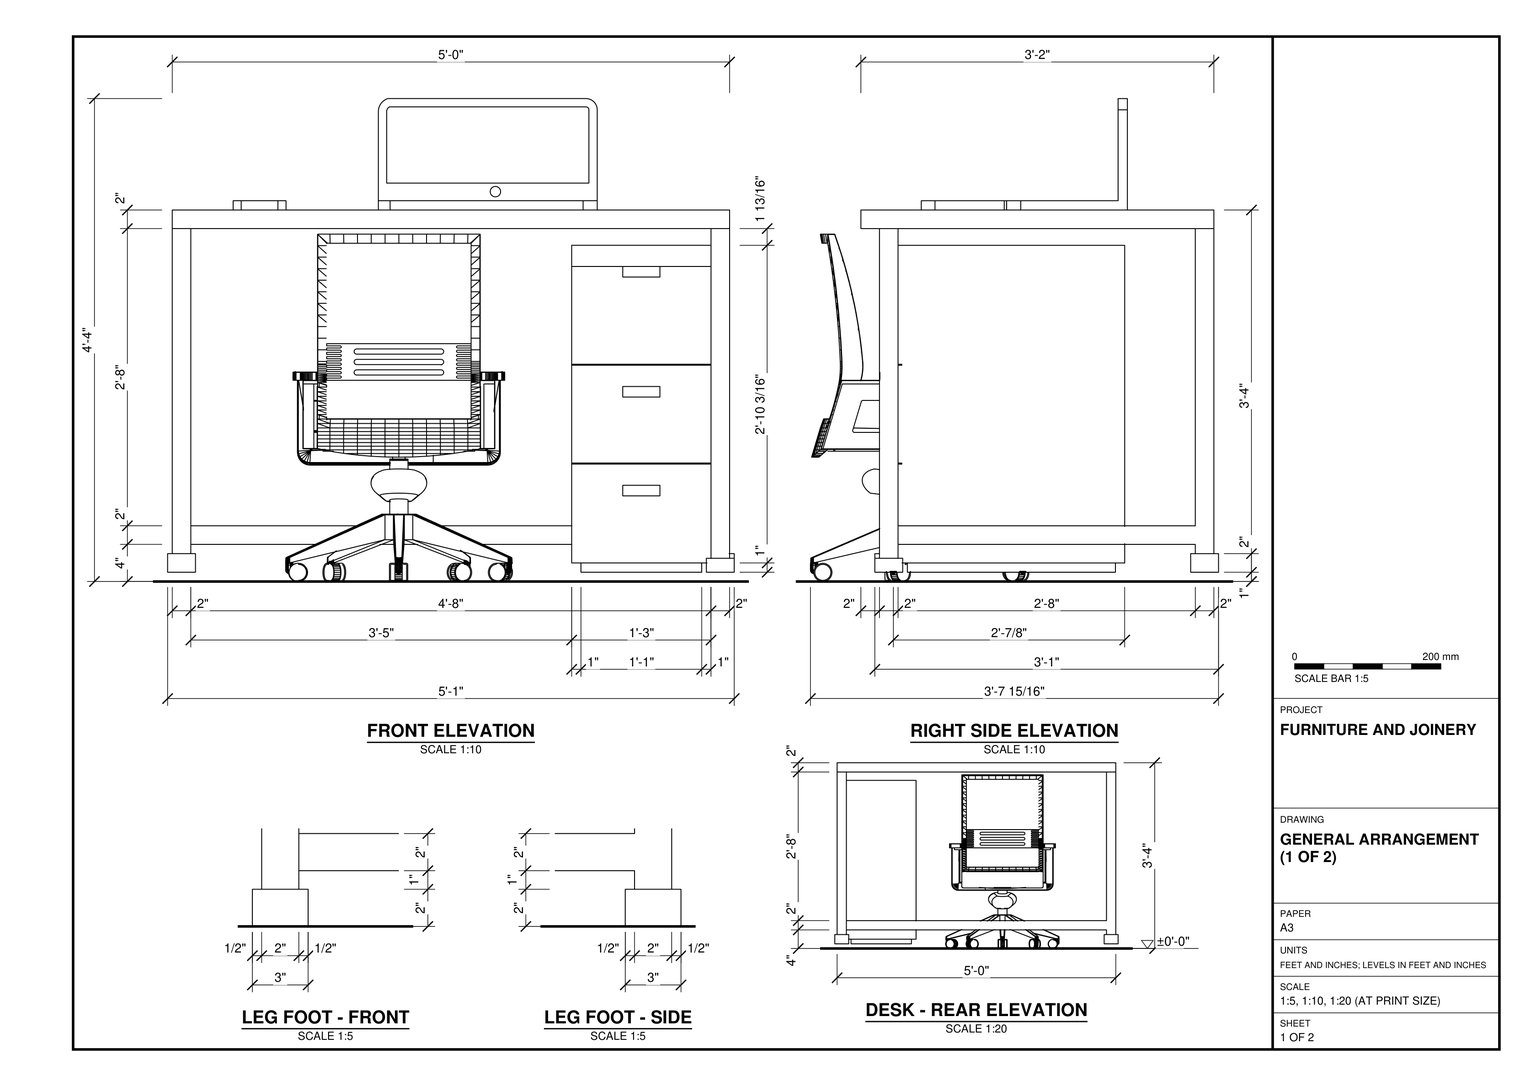
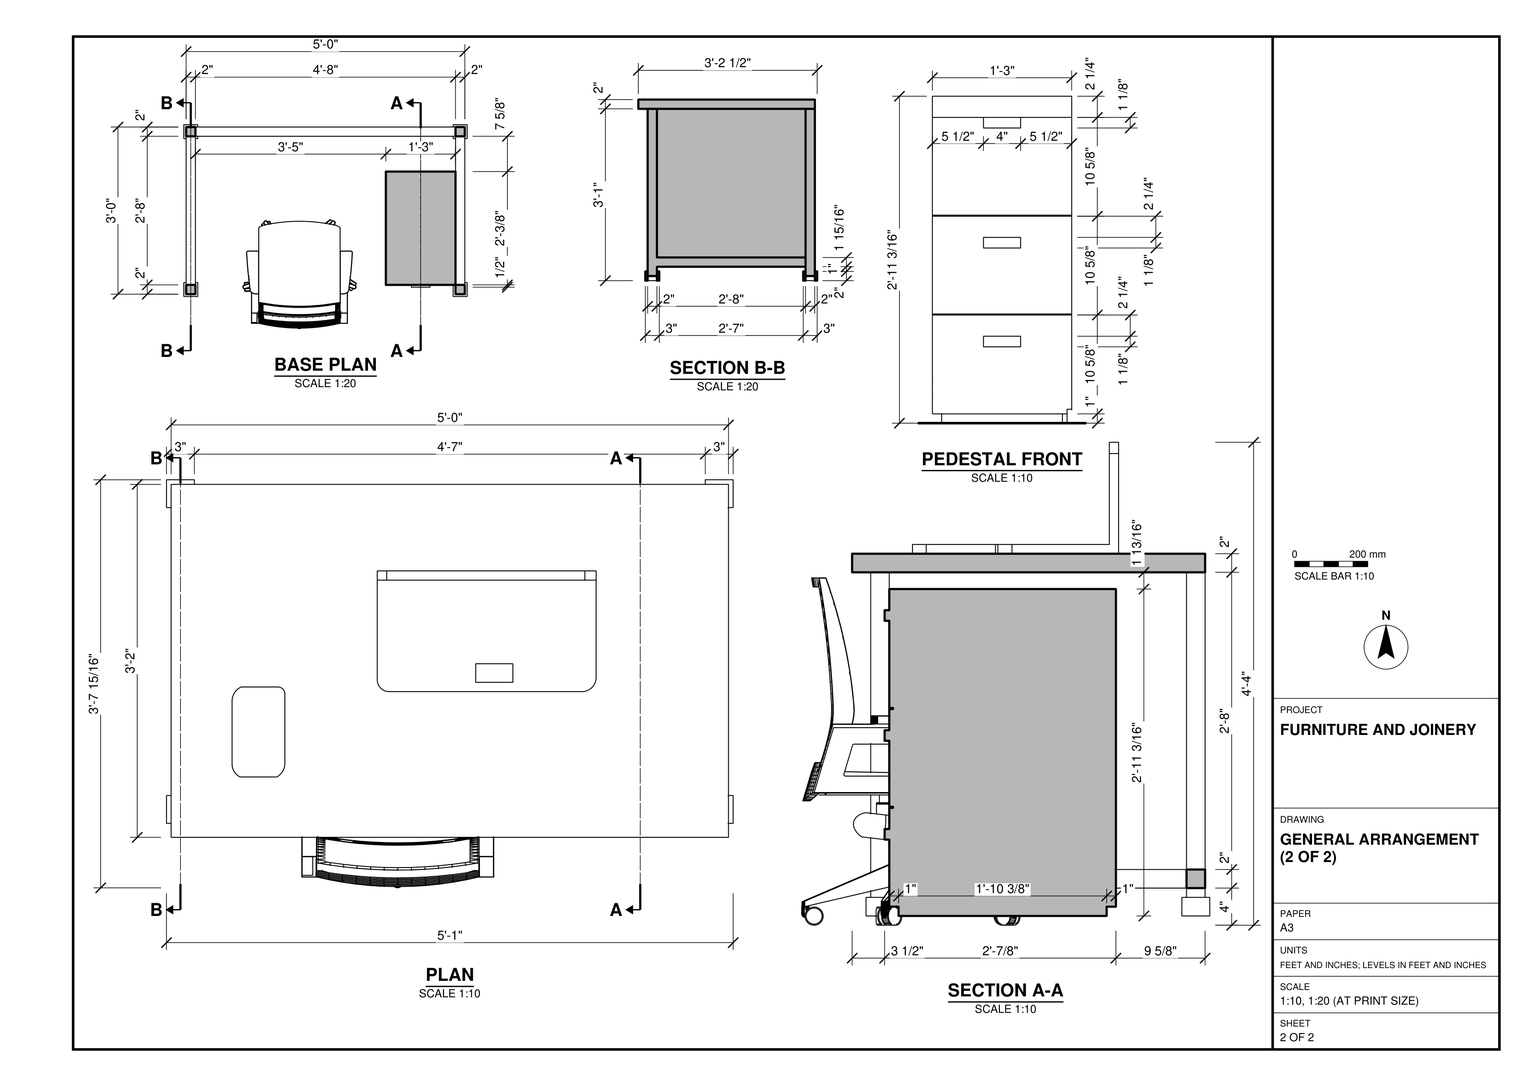
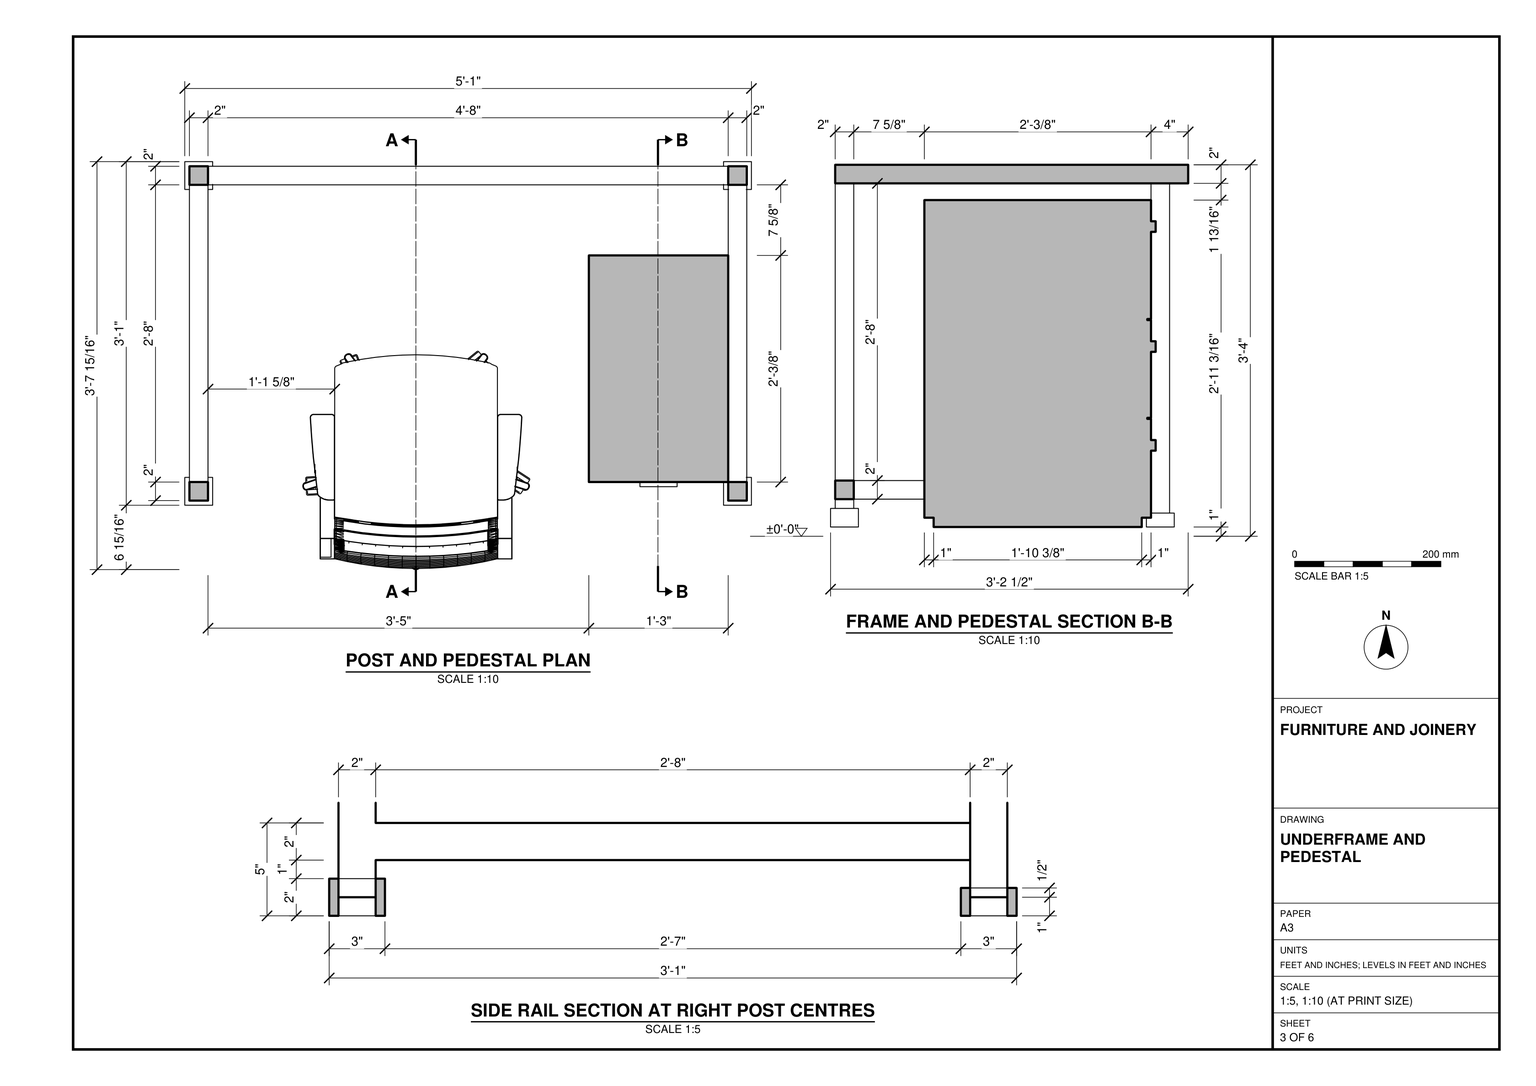
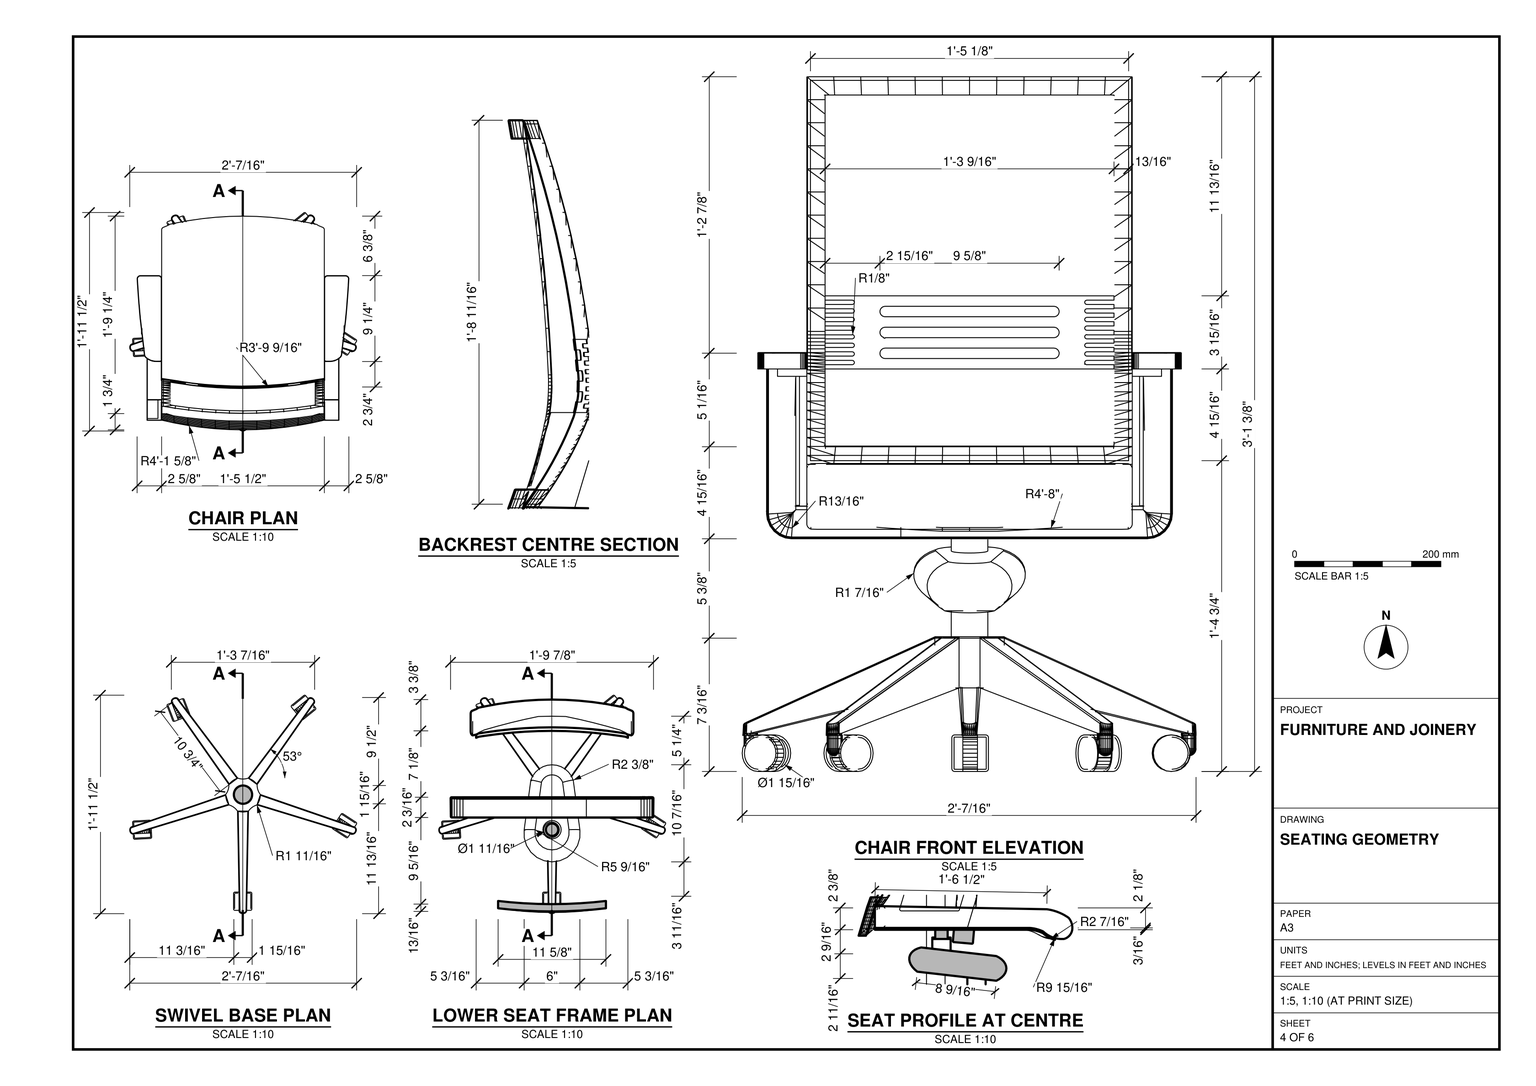
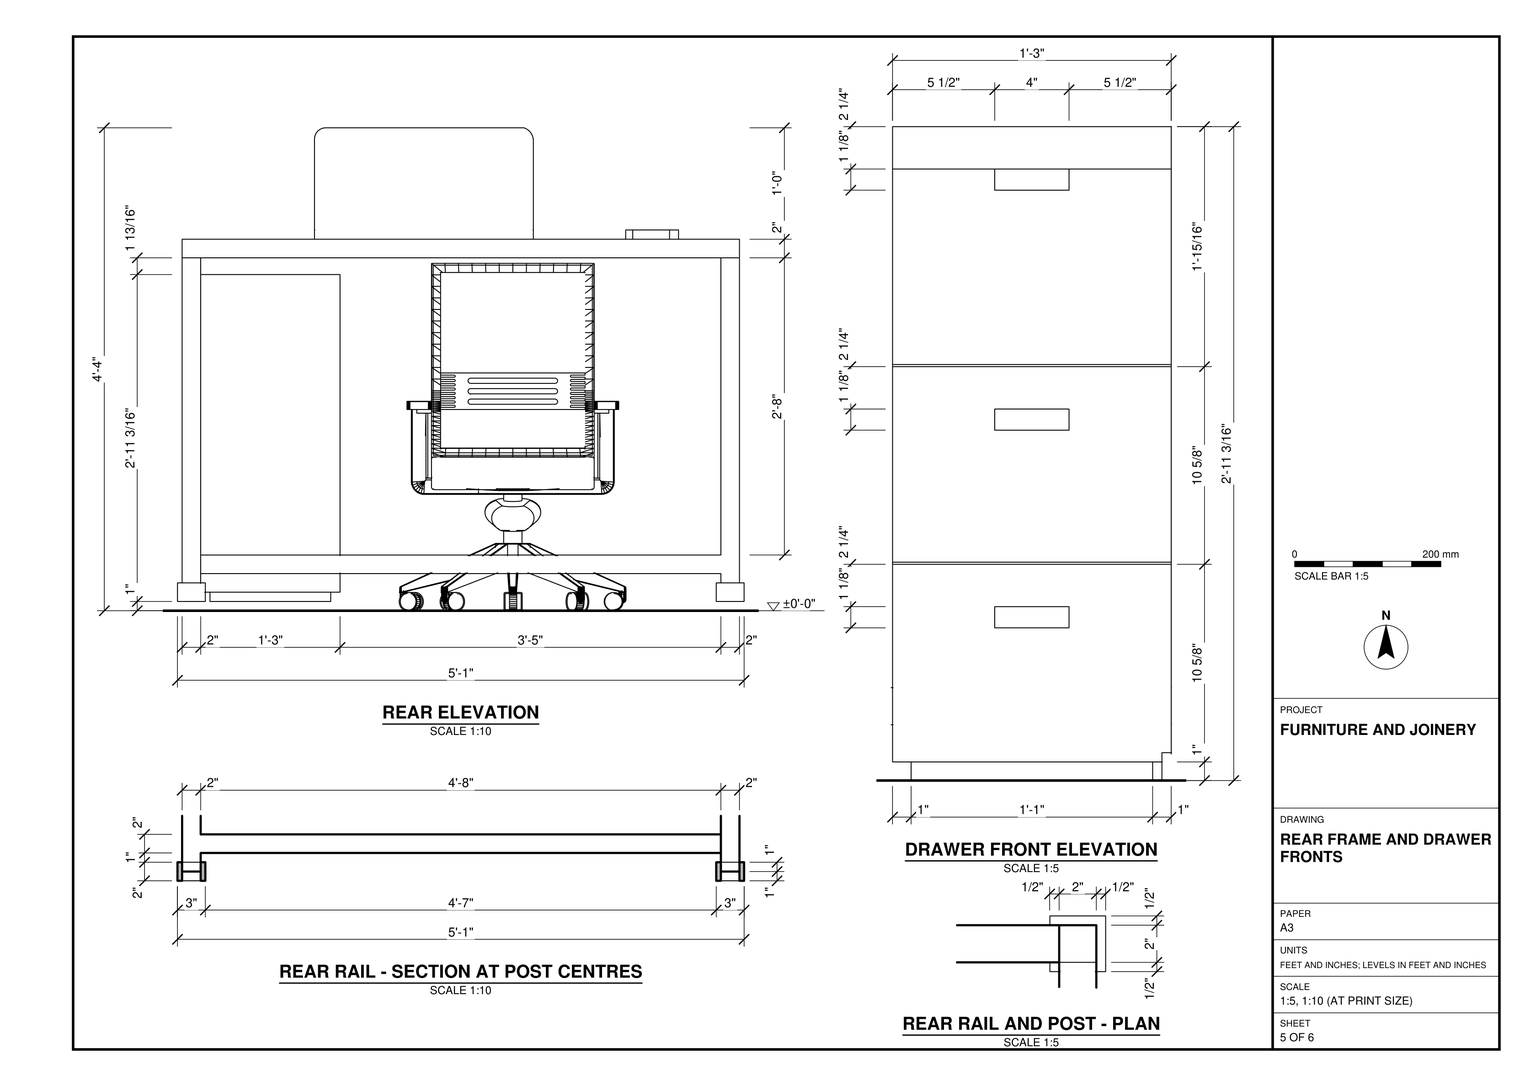
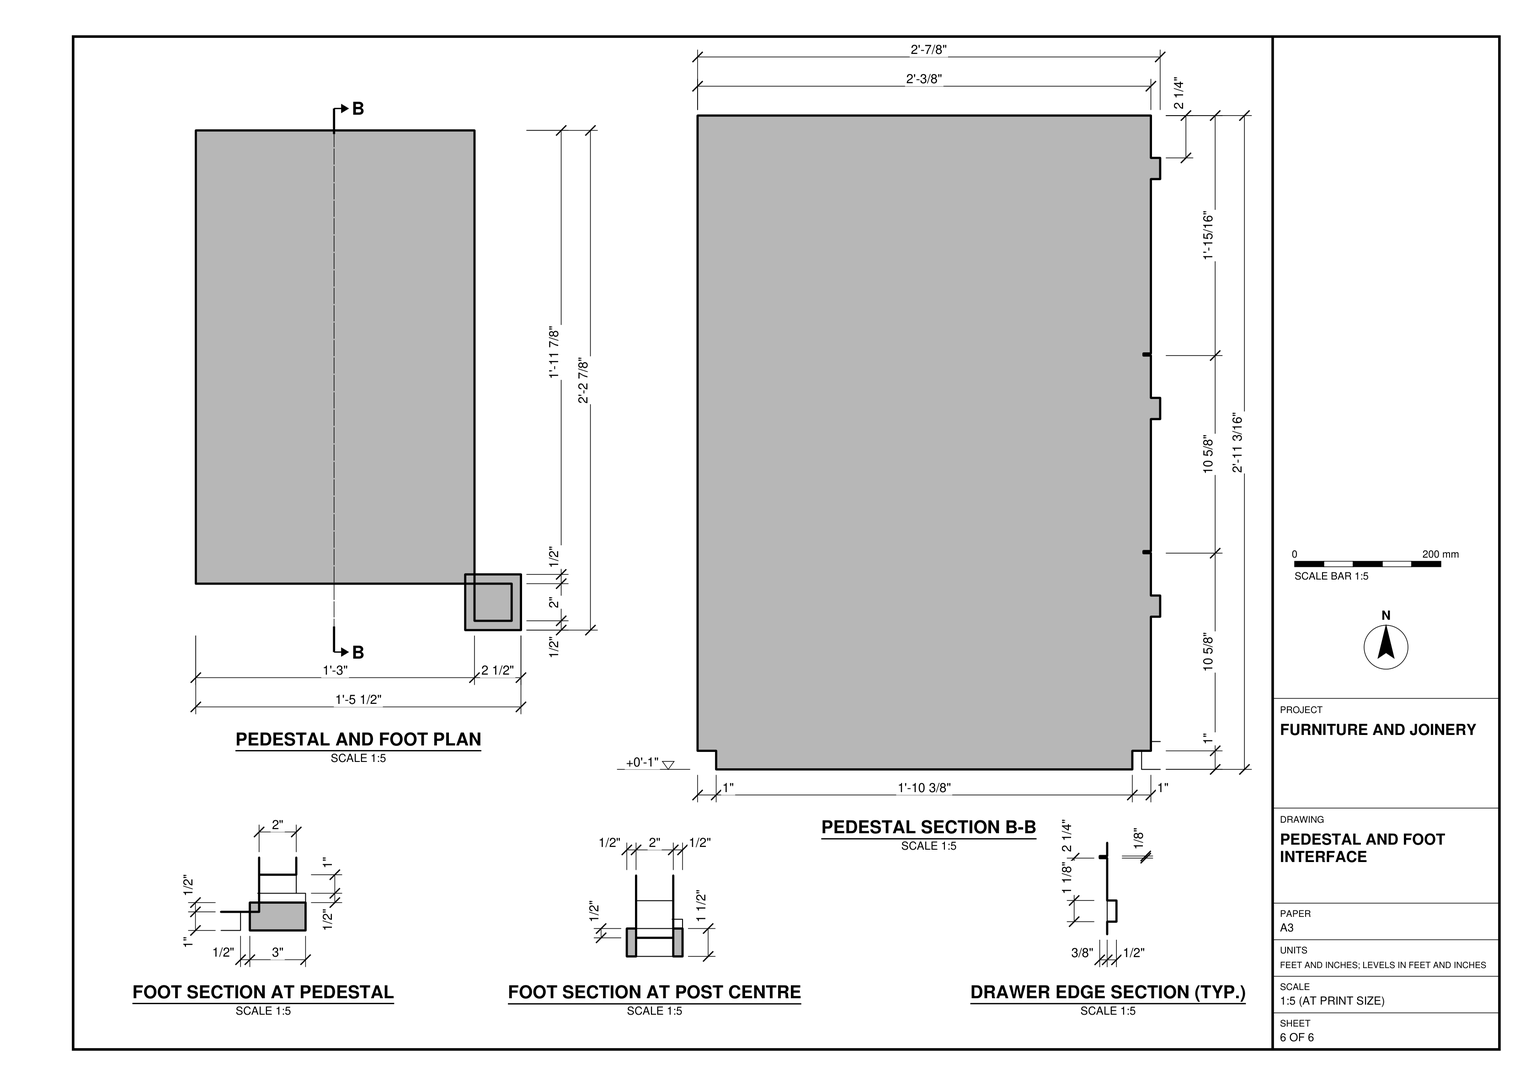
Build the workstation in SketchUp from task_files/diagram_01.pdf. Work in feet and inches, using the floor level marked ±0'-0" as the datum. The complete arrangement, including the chair and the computer, measures 5'-1" wide, 3'-7 15/16" deep and 4'-4" high. Use the front elevation to orient the desk: the drawers face the seated user and are on the right.

Make the rectangular desktop 5'-0" wide, 3'-2" deep and 2" thick. Support it on square corner posts with projecting feet. Connect the posts with low rails along the sides and back, leaving the front of the seating bay open. Fit the drawer pedestal beneath the right end, with a recessed plinth, three stacked drawer fronts and a horizontal pull on each front. Position the armchair on its wheeled base in the open bay, with its back projecting beyond the front feet as shown in plan. Place the computer and the smaller loose item on the desktop in their drawn positions. Decor and loose items may be any suitable library components.

Keep the desk, pedestal, chair and desktop items separately editable as groups or components, and use components for repeated parts. Save one SketchUp model as output_files/workstation_with_a_drawer_pedestal_and_swivel_chair.skp.

# SketchUp Ruby script. Lengths in inches.
U = 1.inch
M = Sketchup.active_model
def pt(a) = Geom::Point3d.new(a.map { |v| v * U })
def face(e, loops, mat)
  f = e.add_face(loops[0].map { |a| pt(a) })
  loops[1..].each { |l| e.add_face(l.map { |a| pt(a) }).erase! }
  f.material = f.back_material = mat if mat
  f
end
# faces: each face lists its corners as indices into pts; further lists are holes
def faces(e, pts, list, mat = nil) = list.each { |f| face(e, (f[0].is_a?(Array) ? f : [f]).map { |l| l.map { |i| pts[i] } }, mat) }
# xy, xz, yz: faces in a plane at the given z, y or x. An outline is a flat list of corners, or four numbers for a rectangle; further outlines are holes
def ring(l) = l.size == 4 ? [[l[0], l[1]], [l[2], l[1]], [l[2], l[3]], [l[0], l[3]]] : l.each_slice(2).to_a
def flat(e, list, mat, &to3) = list.each { |f| face(e, (f[0].is_a?(Array) ? f : [f]).map { |l| ring(l).map { |u, v| to3.(u, v) } }, mat) }
def xy(e, z, list, mat = nil) = flat(e, list, mat) { |x, y| [x, y, z] }
def xz(e, y, list, mat = nil) = flat(e, list, mat) { |x, z| [x, y, z] }
def yz(e, x, list, mat = nil) = flat(e, list, mat) { |y, z| [x, y, z] }
def lines(e, pts, list) = list.each { |a, b| e.add_line(pt(pts[a]), pt(pts[b])) }
# prism: a flat outline (further loops are holes) pulled along v
def prism(e, loops, v, mat = nil)
  f = face(e, loops, mat); d = Geom::Vector3d.new(v.map { |x| x * U })
  f.pushpull(f.normal.samedirection?(d) ? d.length : -d.length)
end
def box(e, o, s, mat = nil) = prism(e, [[o, [o[0] + s[0], o[1], o[2]], [o[0] + s[0], o[1] + s[1], o[2]], [o[0], o[1] + s[1], o[2]]]], [0, 0, s[2]], mat)
def at(x, y, z, deg = 0) = Geom::Transformation.translation(pt([x, y, z])) * Geom::Transformation.rotation(ORIGIN, Z_AXIS, deg.degrees)
def axes(o, x, y, z) = Geom::Transformation.new([*x, 0, *y, 0, *z, 0, *pt(o).to_a, 1])
def part(name) = M.definitions.add(name)
# library, detail: a bought-in or finely detailed component or shape, given as its bounding box
def library(name, o, s) = part(name).tap { |d| box(d.entities, o, s) }
def detail(e, o, s) = box(e.add_group.entities, o, s)
def put(e, d, t, mat = nil) = e.add_instance(d, t).tap { |i| i.material = mat if mat }
def group(e, t, mat = nil) = e.add_group.tap { |g| g.transformation = t; g.material = mat if mat }.entities
root = M.entities
M.materials.add("[Aluminum]").color = [179, 179, 179]
M.materials.add("[Color M07]").color = [58, 58, 58]
M.materials.add("[Metal Seamed]").color = [118, 119, 115]
c1 = library("Office chair",[-0.35,-0.28,0],[24.95,23.8,37.4])
put(root,c1,at(37.14,18.09,0,180))
g1 = group(root,at(0.5,2,2),"[Aluminum]")
g2 = group(g1,at(0,0,0))
xy(g2,-1,[[[-0.5,-0.5,2.5,2.5],[0,0,2,2]]],"[Color M07]")
xy(g2,0,[[0,0,2,2]],"[Color M07]")
xy(g2,1,[[[-0.5,-0.5,2.5,2.5],[0,0,2,2]]],"[Color M07]")
xy(g2,2,[[0,2,2,34]])
xy(g2,4,[[0,2,2,34]])
xy(g2,36,[[0,0,2,2]])
xz(g2,-0.5,[[-0.5,-1,2.5,1]],"[Color M07]")
xz(g2,0,[[0,0,2,1],[0,1,2,36]])
xz(g2,0,[[0,-1,2,0]],"[Color M07]")
xz(g2,2,[[0,0,2,1],[0,1,2,2],[0,4,2,36]])
xz(g2,2,[[0,-1,2,0]],"[Color M07]")
xz(g2,2.5,[[-0.5,-1,2.5,1]],"[Color M07]")
xz(g2,34,[[0,2,2,4]])
yz(g2,-0.5,[[-0.5,-1,2.5,1]],"[Color M07]")
yz(g2,0,[[0,0,2,1],[0,1,0,36,2,36,2,4,34,4,34,2,2,2,2,1]])
yz(g2,0,[[0,-1,2,0]],"[Color M07]")
yz(g2,2,[[0,0,2,1],[0,1,2,1,2,2,34,2,34,4,2,4,2,36,0,36]])
yz(g2,2,[[0,-1,2,0]],"[Color M07]")
yz(g2,2.5,[[-0.5,-1,2.5,1]],"[Color M07]")
g3 = group(g1,at(0,0,36))
box(g3,[0,-2,0],[60,38,2])
g4 = group(g1,at(58,34,0))
xy(g4,-1,[[[-0.5,-0.5,2.5,2.5],[0,0,2,2]]],"[Color M07]")
xy(g4,0,[[0,0,2,2]],"[Color M07]")
xy(g4,1,[[[-0.5,-0.5,2.5,2.5],[0,0,2,2]]],"[Color M07]")
xy(g4,2,[[0,-32,2,0]])
xy(g4,4,[[0,-32,2,0]])
xy(g4,36,[[0,0,2,2]])
xz(g4,-32,[[0,2,2,4]])
xz(g4,-0.5,[[-0.5,-1,2.5,1]],"[Color M07]")
xz(g4,0,[[0,0,2,1],[0,1,2,2],[0,4,2,36]])
xz(g4,0,[[0,-1,2,0]],"[Color M07]")
xz(g4,2,[[0,0,2,1],[0,1,2,36]])
xz(g4,2,[[0,-1,2,0]],"[Color M07]")
xz(g4,2.5,[[-0.5,-1,2.5,1]],"[Color M07]")
yz(g4,-0.5,[[-0.5,-1,2.5,1]],"[Color M07]")
yz(g4,0,[[0,0,2,1],[0,1,0,2,-32,2,-32,4,0,4,0,36,2,36,2,1]])
yz(g4,0,[[0,-1,2,0]],"[Color M07]")
yz(g4,2,[[0,0,2,1],[0,1,2,1,2,36,0,36,0,4,-32,4,-32,2,0,2]])
yz(g4,2,[[0,-1,2,0]],"[Color M07]")
yz(g4,2.5,[[-0.5,-1,2.5,1]],"[Color M07]")
g5 = group(g1,at(58,0,0))
xy(g5,-1,[[[-0.5,-0.5,2.5,2.5],[0,0,2,2]]],"[Color M07]")
xy(g5,0,[[0,0,2,2]],"[Color M07]")
xy(g5,0.5,[[[-0.5,-0.5,2.5,2.5],[0,0,2,2]]],"[Color M07]")
xy(g5,36,[[0,0,2,2]])
xz(g5,-0.5,[[-0.5,-1,2.5,0.5]],"[Color M07]")
xz(g5,0,[[0,0,2,0.5],[0,0.5,2,36]])
xz(g5,0,[[0,-1,2,0]],"[Color M07]")
xz(g5,2,[[0,0,2,0.5],[0,0.5,2,36]])
xz(g5,2,[[0,-1,2,0]],"[Color M07]")
xz(g5,2.5,[[-0.5,-1,2.5,0.5]])
yz(g5,-0.5,[[-0.5,-1,2.5,0.5]],"[Color M07]")
yz(g5,0,[[0,0,2,0.5],[0,0.5,2,36]])
yz(g5,0,[[0,-1,2,0]],"[Color M07]")
yz(g5,2,[[0,0,2,0.5],[0,0.5,2,36]])
yz(g5,2,[[0,-1,2,0]],"[Color M07]")
yz(g5,2.5,[[-0.5,-1,2.5,0.5]],"[Color M07]")
g6 = group(g1,at(0,34,0))
xy(g6,-1,[[[-0.5,-0.5,2.5,2.5],[0,0,2,2]]],"[Color M07]")
xy(g6,0,[[0,0,2,2]],"[Color M07]")
xy(g6,1,[[[-0.5,-0.5,2.5,2.5],[0,0,2,2]]],"[Color M07]")
xy(g6,2,[[2,0,58,2]])
xy(g6,4,[[2,0,58,2]])
xy(g6,36,[[0,0,2,2]])
xz(g6,-0.5,[[-0.5,-1,2.5,1]],"[Color M07]")
xz(g6,0,[[0,0,2,1],[0,1,2,1,2,2,58,2,58,4,2,4,2,36,0,36]])
xz(g6,0,[[0,-1,2,0]],"[Color M07]")
xz(g6,2,[[0,0,2,1],[0,1,0,36,2,36,2,4,58,4,58,2,2,2,2,1]])
xz(g6,2,[[0,-1,2,0]],"[Color M07]")
xz(g6,2.5,[[-0.5,-1,2.5,1]],"[Color M07]")
yz(g6,-0.5,[[-0.5,-1,2.5,1]],"[Color M07]")
yz(g6,0,[[0,0,2,1],[0,1,2,36]])
yz(g6,0,[[0,-1,2,0]],"[Color M07]")
yz(g6,2,[[0,0,2,1],[0,1,2,2],[0,4,2,36]])
yz(g6,2,[[0,-1,2,0]],"[Color M07]")
yz(g6,2.5,[[-0.5,-1,2.5,1]],"[Color M07]")
yz(g6,58,[[0,2,2,4]])
g7 = group(root,at(43.5,3,2),"[Metal Seamed]")
xy(g7,-1,[[1,2,14,24.4]])
xy(g7,0,[[[0,1,15,25.4],[1,2,14,24.4]]])
xy(g7,7.22,[[5.5,0.5,9.5,1]])
xy(g7,8.36,[[5.5,0.5,9.5,1]])
xy(g7,10.64,[[0,1,15,1.4]])
xy(g7,10.75,[[0,1,15,1.4]])
xy(g7,17.86,[[5.5,0.5,9.5,1]])
xy(g7,19,[[5.5,0.5,9.5,1]])
xy(g7,21.28,[[0,1,15,1.4]])
xy(g7,21.39,[[0,1,15,1.4]])
xy(g7,30.78,[[5.5,0.5,9.5,1]])
xy(g7,31.92,[[5.5,0.5,9.5,1]])
xy(g7,34.2,[[0,1,15,25.4]])
xz(g7,0.5,[[5.5,7.22,9.5,8.36],[5.5,17.86,9.5,19],[5.5,30.78,9.5,31.92]])
xz(g7,1,[[[0,0,15,10.64],[5.5,7.22,9.5,8.36]],[[0,10.75,15,21.28],[5.5,17.86,9.5,19]],[0,21.39,15,21.39,15,31.92,9.5,31.92,9.5,30.78,5.5,30.78,5.5,31.92,0,31.92],[0,31.92,15,34.2]])
xz(g7,1.4,[[0,10.64,15,10.75],[0,21.28,15,21.39]])
xz(g7,2,[[1,-1,14,0]])
xz(g7,24.4,[[1,-1,14,0]])
xz(g7,25.4,[[0,0,15,34.2]])
yz(g7,0,[[1,0,1,10.64,1.4,10.64,1.4,10.75,1,10.75,1,21.28,1.4,21.28,1.4,21.39,1,21.39,1,34.2,25.4,34.2,25.4,0]])
yz(g7,1,[[2,-1,24.4,0]])
yz(g7,5.5,[[0.5,7.22,1,8.36],[0.5,17.86,1,19],[0.5,30.78,1,31.92]])
yz(g7,9.5,[[0.5,7.22,1,8.36],[0.5,17.86,1,19],[0.5,30.78,1,31.92]])
yz(g7,14,[[2,-1,24.4,0]])
yz(g7,15,[[1,0,25.4,0,25.4,34.2,1,34.2,1,21.39,1.4,21.39,1.4,21.28,1,21.28,1,10.75,1.4,10.75,1.4,10.64,1,10.64]])
g8 = group(root,at(7.06,6.5,40))
prism(g8,[[[0,1.38,0],[0,8.16,0],[0.01,8.32,0],[0.03,8.48,0],[0.07,8.63,0],[0.12,8.78,0],[0.18,8.93,0],[0.26,9.06,0],[0.35,9.19,0],[0.46,9.32,0],[0.57,9.43,0],[0.7,9.53,0],[0.83,9.61,0],[0.97,9.6875,0],[4.93,9.6875,0],[5.03,9.68,0],[5.13,9.66,0],[5.22,9.63,0],[5.31,9.59,0],[5.39,9.53,0],[5.47,9.47,0],[5.53,9.39,0],[5.59,9.31,0],[5.63,9.22,0],[5.66,9.13,0],[5.68,9.03,0],[5.6875,8.93,0],[5.6875,1.48,0],[5.68,1.33,0],[5.66,1.18,0],[5.63,1.03,0],[5.58,0.89,0],[5.52,0.75,0],[5.45,0.62,0],[5.375,0.5,0],[5.28,0.38,0],[5.18,0.27,0],[5.07,0.17,0],[4.95,0.08,0],[4.82,0,0],[0.86,0,0],[0.74,0.07,0],[0.62,0.15,0],[0.51,0.24,0],[0.41,0.34,0],[0.31,0.45,0],[0.23,0.57,0],[0.16,0.69,0],[0.11,0.82,0],[0.06,0.96,0],[0.03,1.1,0],[0.01,1.24,0]]],[0,0,1])
g9 = group(root,at(22.6875,15.6875,40))
xy(g9,0,[[1.27,0,1.1,0.01,0.9375,0.04,0.78,0.1,0.63,0.17,0.5,0.26,0.37,0.37,0.26,0.5,0.17,0.63,0.1,0.78,0.04,0.9375,0.01,1.1,0,1.27,0,13,23.5625,13,23.5625,1.52,23.55,1.32,23.51,1.125,23.45,0.9375,23.36,0.76,23.25,0.59,23.12,0.45,22.97,0.3125,22.8,0.2,22.625,0.12,22.4375,0.05,22.24,0.01,22.04,0]])
xy(g9,0.9,[[10.6,1,14.6,3]])
xy(g9,1,[[[1.27,0,22.04,0,22.24,0.01,22.4375,0.05,22.625,0.12,22.8,0.2,22.97,0.3125,23.12,0.45,23.25,0.59,23.36,0.76,23.45,0.9375,23.51,1.125,23.55,1.32,23.5625,1.52,23.5625,12,0,12,0,1.27,0.01,1.1,0.04,0.9375,0.1,0.78,0.17,0.63,0.26,0.5,0.37,0.37,0.5,0.26,0.63,0.17,0.78,0.1,0.9375,0.04,1.1,0.01],[10.6,1,14.6,3]]])
xy(g9,12,[[1.02,12,22.35,13]])
xz(g9,0,[[1.27,0,22.04,1]])
xz(g9,1,[[10.6,0.9,14.6,1]])
xz(g9,3,[[10.6,0.9,14.6,1]])
xz(g9,12,[[[0,1,23.5625,1,23.5625,10.79,23.55,10.95,23.52,11.1,23.47,11.25,23.4,11.39,23.3125,11.53,23.21,11.64,23.09,11.75,22.96,11.84,22.8125,11.91,22.66,11.96,22.51,11.99,22.35,12,1.02,12,0.875,11.94,0.74,11.875,0.61,11.79,0.49,11.69,0.38,11.59,0.28,11.47,0.2,11.34,0.13,11.2,0.07,11.05,0.03,10.91,0.01,10.75,0,10.6],[0.9,2.9,0.9,10.66,0.92,10.78,0.95,10.83,0.97,10.89,1.01,10.9375,1.04,10.98,1.13,11.07,1.18,11.1,22.39,11.1,22.47,11.08,22.51,11.0625,22.54,11.04,22.6,10.98,22.625,10.95,22.64,10.91,22.66,10.87,22.66,10.83,22.67,10.79,22.67,2.9],[12.55,1.42,12.4,1.45,12.28,1.52,12.17,1.62,12.09,1.74,12.05,1.88,12.04,2.03,12.07,2.17,12.14,2.3,12.24,2.41,12.37,2.49,12.51,2.53,12.66,2.54,12.8,2.5,12.93,2.4375,13.04,2.34,13.11,2.21,13.16,2.07,13.16,1.92,13.13,1.78,13.06,1.65,12.96,1.54,12.84,1.47,12.69,1.42]],[12.55,1.42,12.69,1.42,12.84,1.47,12.96,1.54,13.06,1.65,13.13,1.78,13.16,1.92,13.16,2.07,13.11,2.21,13.04,2.34,12.93,2.4375,12.8,2.5,12.66,2.54,12.51,2.53,12.37,2.49,12.24,2.41,12.14,2.3,12.07,2.17,12.04,2.03,12.05,1.88,12.09,1.74,12.17,1.62,12.28,1.52,12.4,1.45],[0.9,2.9,22.67,2.9,22.67,10.79,22.66,10.83,22.66,10.87,22.64,10.91,22.625,10.95,22.6,10.98,22.54,11.04,22.51,11.0625,22.47,11.08,22.39,11.1,1.18,11.1,1.13,11.07,1.04,10.98,1.01,10.9375,0.97,10.89,0.95,10.83,0.92,10.78,0.9,10.66]])
xz(g9,13,[[0,0,0,10.6,0.01,10.75,0.03,10.91,0.07,11.05,0.13,11.2,0.2,11.34,0.28,11.47,0.38,11.59,0.49,11.69,0.61,11.79,0.74,11.875,0.875,11.94,1.02,12,22.35,12,22.51,11.99,22.66,11.96,22.8125,11.91,22.96,11.84,23.09,11.75,23.21,11.64,23.3125,11.53,23.4,11.39,23.47,11.25,23.52,11.1,23.55,10.95,23.5625,10.79,23.5625,0]])
yz(g9,0,[[1.27,0,1.27,1,12,1,12,10.6,13,10.6,13,0]])
yz(g9,10.6,[[1,0.9,3,1]])
yz(g9,14.6,[[1,0.9,3,1]])
yz(g9,23.5625,[[1.52,0,13,0,13,10.79,12,10.79,12,1,1.52,1]])
p = [[0.9375,0.04,1],[0.78,0.1,1],[0.78,0.1,0],[0.9375,0.04,0],[1.1,0.01,1],[1.1,0.01,0],
  [1.27,0,1],[1.27,0,0],[22.24,0.01,1],[22.04,0,1],[22.04,0,0],[22.24,0.01,0],
  [22.4375,0.05,1],[22.4375,0.05,0],[0.63,0.17,1],[0.63,0.17,0],[22.625,0.12,1],[22.625,0.12,0],
  [22.8,0.2,1],[22.8,0.2,0],[0.5,0.26,1],[0.5,0.26,0],[22.97,0.3125,1],[22.97,0.3125,0],
  [0.37,0.37,1],[0.37,0.37,0],[23.12,0.45,1],[23.12,0.45,0],[0.26,0.5,1],[0.26,0.5,0],
  [23.25,0.59,1],[23.25,0.59,0],[0.17,0.63,1],[0.17,0.63,0],[0.1,0.78,1],[0.1,0.78,0],
  [23.36,0.76,1],[23.36,0.76,0],[0.04,0.9375,1],[0.04,0.9375,0],[23.45,0.9375,1],[23.45,0.9375,0],
  [0.01,1.1,1],[0.01,1.1,0],[23.51,1.125,1],[23.51,1.125,0],[0,1.27,1],[0,1.27,0],
  [23.55,1.32,1],[23.55,1.32,0],[23.5625,1.52,1],[23.5625,1.52,0],[0,12,10.6],[0.01,12,10.75],
  [0.01,13,10.75],[0,13,10.6],[0.03,12,10.91],[0.03,13,10.91],[23.55,12,10.95],[23.5625,12,10.79],
  [23.5625,13,10.79],[23.55,13,10.95],[0.07,12,11.05],[0.07,13,11.05],[23.52,12,11.1],[23.52,13,11.1],
  [0.13,12,11.2],[0.13,13,11.2],[23.47,12,11.25],[23.47,13,11.25],[0.2,12,11.34],[0.2,13,11.34],
  [0.28,12,11.47],[0.28,13,11.47],[23.4,12,11.39],[23.4,13,11.39],[23.3125,12,11.53],[23.3125,13,11.53],
  [0.38,12,11.59],[0.38,13,11.59],[23.21,12,11.64],[23.21,13,11.64],[0.49,12,11.69],[0.49,13,11.69],
  [23.09,12,11.75],[23.09,13,11.75],[0.61,12,11.79],[0.61,13,11.79],[22.96,12,11.84],[22.96,13,11.84],
  [0.74,12,11.875],[0.74,13,11.875],[22.8125,12,11.91],[22.8125,13,11.91],[0.875,12,11.94],[0.875,13,11.94],
  [1.02,12,12],[1.02,13,12],[22.66,12,11.96],[22.66,13,11.96],[22.35,12,12],[22.51,12,11.99],
  [22.51,13,11.99],[22.35,13,12]]
faces(g9,p,[[0,1,2,3],[4,0,3,5],[6,4,5,7],[8,9,10,11],[12,8,11,13],[1,14,15,2],[16,12,13,17],[18,16,17,19],
  [14,20,21,15],[22,18,19,23],[20,24,25,21],[26,22,23,27],[24,28,29,25],[30,26,27,31],[28,32,33,29],[32,34,35,33],
  [36,30,31,37],[34,38,39,35],[40,36,37,41],[38,42,43,39],[44,40,41,45],[42,46,47,43],[48,44,45,49],[50,48,49,51],
  [52,53,54,55],[53,56,57,54],[58,59,60,61],[56,62,63,57],[64,58,61,65],[62,66,67,63],[68,64,65,69],[66,70,71,67],
  [70,72,73,71],[74,68,69,75],[76,74,75,77],[72,78,79,73],[80,76,77,81],[78,82,83,79],[84,80,81,85],[82,86,87,83],
  [88,84,85,89],[86,90,91,87],[92,88,89,93],[90,94,95,91],[94,96,97,95],[98,92,93,99],[100,101,102,103],[101,98,99,102]])
